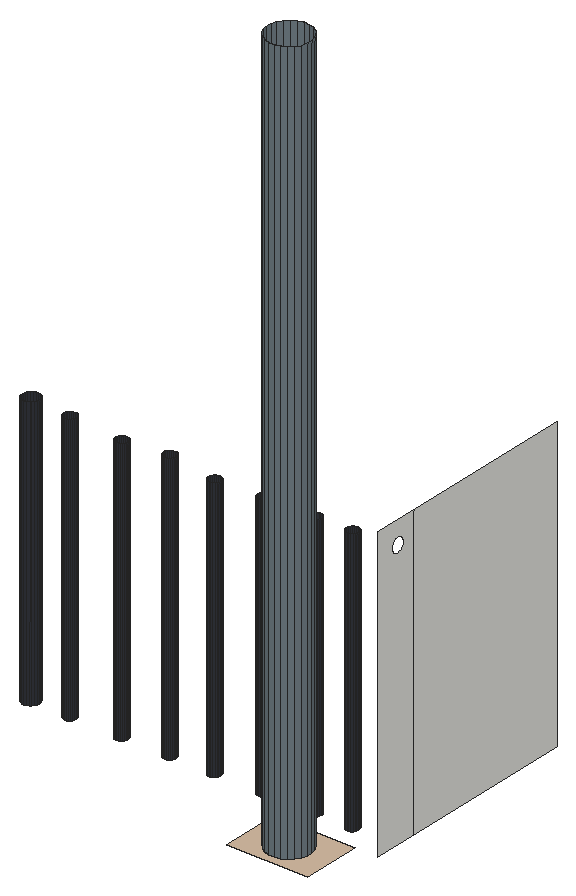
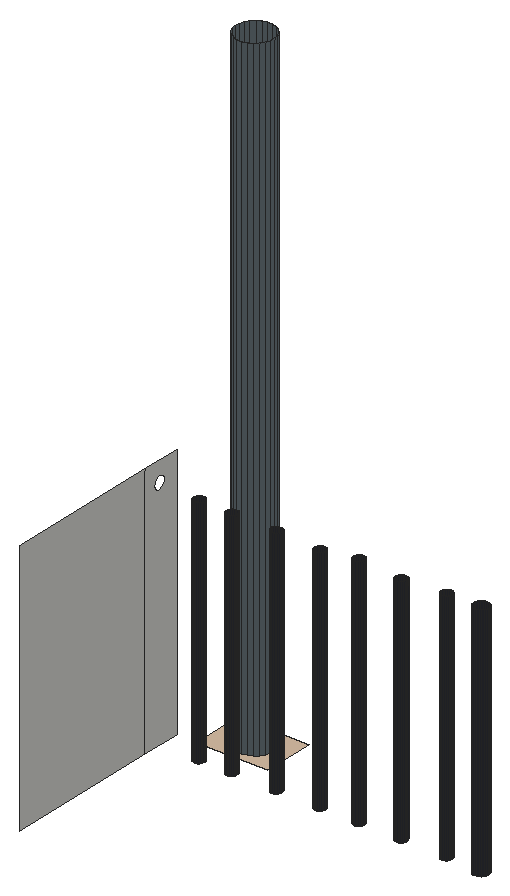
# SketchUp Ruby script. Lengths in inches.
U = 1.inch
M = Sketchup.active_model
def pt(a) = Geom::Point3d.new(a.map { |v| v * U })
def face(e, loops, mat)
  f = e.add_face(loops[0].map { |a| pt(a) })
  loops[1..].each { |l| e.add_face(l.map { |a| pt(a) }).erase! }
  f.material = f.back_material = mat if mat
  f
end
# faces: each face lists its corners as indices into pts; further lists are holes
def faces(e, pts, list, mat = nil) = list.each { |f| face(e, (f[0].is_a?(Array) ? f : [f]).map { |l| l.map { |i| pts[i] } }, mat) }
# xy, xz, yz: faces in a plane at the given z, y or x. An outline is a flat list of corners, or four numbers for a rectangle; further outlines are holes
def ring(l) = l.size == 4 ? [[l[0], l[1]], [l[2], l[1]], [l[2], l[3]], [l[0], l[3]]] : l.each_slice(2).to_a
def flat(e, list, mat, &to3) = list.each { |f| face(e, (f[0].is_a?(Array) ? f : [f]).map { |l| ring(l).map { |u, v| to3.(u, v) } }, mat) }
def xy(e, z, list, mat = nil) = flat(e, list, mat) { |x, y| [x, y, z] }
def xz(e, y, list, mat = nil) = flat(e, list, mat) { |x, z| [x, y, z] }
def yz(e, x, list, mat = nil) = flat(e, list, mat) { |y, z| [x, y, z] }
def lines(e, pts, list) = list.each { |a, b| e.add_line(pt(pts[a]), pt(pts[b])) }
# prism: a flat outline (further loops are holes) pulled along v
def prism(e, loops, v, mat = nil)
  f = face(e, loops, mat); d = Geom::Vector3d.new(v.map { |x| x * U })
  f.pushpull(f.normal.samedirection?(d) ? d.length : -d.length)
end
def box(e, o, s, mat = nil) = prism(e, [[o, [o[0] + s[0], o[1], o[2]], [o[0] + s[0], o[1] + s[1], o[2]], [o[0], o[1] + s[1], o[2]]]], [0, 0, s[2]], mat)
def at(x, y, z, deg = 0) = Geom::Transformation.translation(pt([x, y, z])) * Geom::Transformation.rotation(ORIGIN, Z_AXIS, deg.degrees)
def axes(o, x, y, z) = Geom::Transformation.new([*x, 0, *y, 0, *z, 0, *pt(o).to_a, 1])
def part(name) = M.definitions.add(name)
# library, detail: a bought-in or finely detailed component or shape, given as its bounding box
def library(name, o, s) = part(name).tap { |d| box(d.entities, o, s) }
def detail(e, o, s) = box(e.add_group.entities, o, s)
def put(e, d, t, mat = nil) = e.add_instance(d, t).tap { |i| i.material = mat if mat }
def group(e, t, mat = nil) = e.add_group.tap { |g| g.transformation = t; g.material = mat if mat }.entities
root = M.entities
M.materials.add("[Formica Laminate Dark]").color = [50, 53, 60]
M.materials.add("[Formica Laminate Light]").color = [213, 189, 164]
M.materials.add("[Formica Speckled Grey]").color = [112, 125, 132]
xy(root,160.3,[[376.35,84.16,375.77,84.33,375.25,84.63,374.83,85.07,374.53,85.59,374.38,86.18,374.39,86.78,374.55,87.36,374.86,87.88,375.29,88.3,375.82,88.6,376.4,88.75,377.01,88.74,377.59,88.58,378.11,88.27,378.53,87.84,378.83,87.3125,378.98,86.73,378.97,86.125,378.81,85.54,378.5,85.02,378.07,84.6,377.54,84.31,376.95,84.16],[343.65,91.54,343.41,91.57,343.18,91.66,342.99,91.8125,342.84,92.01,342.75,92.23,342.71,92.47,342.75,92.72,342.84,92.94,342.99,93.14,343.18,93.29,343.41,93.38,343.65,93.41,343.89,93.38,344.12,93.29,344.31,93.14,344.46,92.94,344.56,92.72,344.59,92.47,344.56,92.23,344.46,92.01,344.31,91.8125,344.12,91.66,343.89,91.57],[348.06,91.61,347.88,91.64,347.72,91.7,347.57,91.8125,347.46,91.96,347.4,92.12,347.37,92.3,347.4,92.48,347.46,92.64,347.57,92.79,347.72,92.89,347.88,92.96,348.06,92.99,348.24,92.96,348.4,92.89,348.55,92.79,348.65,92.64,348.72,92.48,348.75,92.3,348.72,92.12,348.65,91.96,348.55,91.8125,348.4,91.7,348.24,91.64],[353.72,91.61,353.54,91.64,353.375,91.7,353.23,91.8125,353.125,91.96,353.06,92.12,353.03,92.3,353.06,92.48,353.125,92.64,353.23,92.79,353.375,92.89,353.54,92.96,353.72,92.99,353.9,92.96,354.0625,92.89,354.21,92.79,354.32,92.64,354.38,92.48,354.41,92.3,354.38,92.12,354.32,91.96,354.21,91.8125,354.0625,91.7,353.9,91.64],[358.97,91.61,358.79,91.64,358.625,91.7,358.48,91.8125,358.375,91.96,358.31,92.12,358.28,92.3,358.31,92.48,358.375,92.64,358.48,92.79,358.625,92.89,358.79,92.96,358.97,92.99,359.15,92.96,359.3125,92.89,359.46,92.79,359.57,92.64,359.63,92.48,359.66,92.3,359.63,92.12,359.57,91.96,359.46,91.8125,359.3125,91.7,359.15,91.64],
  [363.84,91.61,363.67,91.64,363.5,91.7,363.36,91.8125,363.25,91.96,363.18,92.12,363.16,92.3,363.18,92.48,363.25,92.64,363.36,92.79,363.5,92.89,363.67,92.96,363.84,92.99,364.02,92.96,364.1875,92.89,364.33,92.79,364.44,92.64,364.51,92.48,364.53,92.3,364.51,92.12,364.44,91.96,364.33,91.8125,364.1875,91.7,364.02,91.64],[369.28,91.61,369.1,91.64,368.9375,91.7,368.8,91.8125,368.6875,91.96,368.62,92.12,368.59,92.3,368.62,92.48,368.6875,92.64,368.8,92.79,368.9375,92.89,369.1,92.96,369.28,92.99,369.46,92.96,369.625,92.89,369.77,92.79,369.88,92.64,369.95,92.48,369.97,92.3,369.95,92.12,369.88,91.96,369.77,91.8125,369.625,91.7,369.46,91.64],[374.84,91.61,374.67,91.64,374.5,91.7,374.36,91.8125,374.25,91.96,374.18,92.12,374.16,92.3,374.18,92.48,374.25,92.64,374.36,92.79,374.5,92.89,374.67,92.96,374.84,92.99,375.02,92.96,375.1875,92.89,375.33,92.79,375.44,92.64,375.51,92.48,375.53,92.3,375.51,92.12,375.44,91.96,375.33,91.8125,375.1875,91.7,375.02,91.64],[378.93,91.61,378.76,91.64,378.59,91.7,378.45,91.8125,378.34,91.96,378.27,92.12,378.25,92.3,378.27,92.48,378.34,92.64,378.45,92.79,378.59,92.89,378.76,92.96,378.93,92.99,379.11,92.96,379.28,92.89,379.42,92.79,379.53,92.64,379.6,92.48,379.62,92.3,379.6,92.12,379.53,91.96,379.42,91.8125,379.28,91.7,379.11,91.64]])
xy(root,160.3,[[[372.44,83.29,381.28,89.73],[376.35,84.16,375.77,84.33,375.25,84.63,374.83,85.07,374.53,85.59,374.38,86.18,374.39,86.78,374.55,87.36,374.86,87.88,375.29,88.3,375.82,88.6,376.4,88.75,377.01,88.74,377.59,88.58,378.11,88.27,378.53,87.84,378.83,87.3125,378.98,86.73,378.97,86.125,378.81,85.54,378.5,85.02,378.07,84.6,377.54,84.31,376.95,84.16]]],"[Formica Laminate Light]")
xz(root,84.16,[[376.35,160.3,376.95,239.81]],"[Formica Speckled Grey]")
yz(root,383.79,[[[89.73,160.3,94.63,192.125],[92.39,188.79,92.6,188.82,92.8,188.9,92.96,189.03,93.09,189.2,93.18,189.39,93.2,189.6,93.18,189.8125,93.09,190.01,92.96,190.18,92.8,190.31,92.6,190.39,92.39,190.42,92.18,190.39,91.98,190.31,91.82,190.18,91.6875,190.01,91.61,189.8125,91.58,189.6,91.61,189.39,91.6875,189.2,91.82,189.03,91.98,188.9,92.18,188.82]],[94.63,160.3,114.1,192.125]])
p = [[375.77,84.33,160.3],[376.35,84.16,160.3],[376.35,84.16,239.81],[375.77,84.33,239.81],[376.95,84.16,160.3],[377.54,84.31,160.3],
  [377.54,84.31,239.81],[376.95,84.16,239.81],[375.25,84.63,160.3],[375.25,84.63,239.81],[378.07,84.6,160.3],[378.07,84.6,239.81],
  [374.83,85.07,160.3],[374.83,85.07,239.81],[378.5,85.02,160.3],[378.5,85.02,239.81],[378.81,85.54,160.3],[378.81,85.54,239.81],
  [374.53,85.59,160.3],[374.53,85.59,239.81],[378.97,86.125,160.3],[378.97,86.125,239.81],[374.38,86.18,160.3],[374.38,86.18,239.81],
  [378.98,86.73,160.3],[378.98,86.73,239.81],[374.39,86.78,160.3],[374.39,86.78,239.81],[378.83,87.3125,160.3],[378.83,87.3125,239.81],
  [374.55,87.36,160.3],[374.55,87.36,239.81],[378.53,87.84,160.3],[378.53,87.84,239.81],[374.86,87.88,160.3],[374.86,87.88,239.81],
  [378.11,88.27,160.3],[378.11,88.27,239.81],[375.29,88.3,160.3],[375.29,88.3,239.81],[375.82,88.6,160.3],[375.82,88.6,239.81],
  [377.59,88.58,160.3],[377.59,88.58,239.81],[376.4,88.75,160.3],[376.4,88.75,239.81],[377.01,88.74,160.3],[377.01,88.74,239.81],
  [343.41,91.57,160.3],[343.65,91.54,160.3],[343.65,91.54,190.01],[343.41,91.57,190.01],[343.89,91.57,160.3],[343.89,91.57,190.01],
  [343.18,91.66,160.3],[343.18,91.66,190.01],[344.12,91.66,160.3],[344.12,91.66,190.01],[347.72,91.7,160.3],[347.88,91.64,160.3],
  [347.88,91.64,189.8],[347.72,91.7,189.8],[348.06,91.61,160.3],[348.06,91.61,189.8],[348.24,91.64,160.3],[348.24,91.64,189.8],
  [348.4,91.7,160.3],[348.4,91.7,189.8],[353.375,91.7,160.3],[353.54,91.64,160.3],[353.54,91.64,189.42],[353.375,91.7,189.42],
  [353.72,91.61,160.3],[353.72,91.61,189.42],[353.9,91.64,160.3],[353.9,91.64,189.42],[354.0625,91.7,160.3],[354.0625,91.7,189.42],
  [358.625,91.7,160.3],[358.79,91.64,160.3],[358.79,91.64,189.8125],[358.625,91.7,189.8125],[358.97,91.61,160.3],[358.97,91.61,189.8125],
  [359.15,91.64,160.3],[359.15,91.64,189.8125],[359.3125,91.7,160.3],[359.3125,91.7,189.8125],[363.5,91.7,160.3],[363.67,91.64,160.3],
  [363.67,91.64,189.11],[363.5,91.7,189.11],[363.84,91.61,160.3],[363.84,91.61,189.11],[364.02,91.64,160.3],[364.02,91.64,189.11],
  [364.1875,91.7,160.3],[364.1875,91.7,189.11],[368.9375,91.7,160.3],[369.1,91.64,160.3],[369.1,91.64,189.36],[368.9375,91.7,189.36],
  [369.28,91.61,160.3],[369.28,91.61,189.36],[369.46,91.64,160.3],[369.46,91.64,189.36],[369.625,91.7,160.3],[369.625,91.7,189.36],
  [374.5,91.7,160.3],[374.67,91.64,160.3],[374.67,91.64,189.36],[374.5,91.7,189.36],[374.84,91.61,160.3],[374.84,91.61,189.36],
  [375.02,91.64,160.3],[375.02,91.64,189.36],[375.1875,91.7,160.3],[375.1875,91.7,189.36],[378.59,91.7,160.3],[378.76,91.64,160.3],
  [378.76,91.64,189.42],[378.59,91.7,189.42],[378.93,91.61,160.3],[378.93,91.61,189.42],[379.11,91.64,160.3],[379.11,91.64,189.42],
  [379.28,91.7,160.3],[379.28,91.7,189.42],[342.99,91.8125,160.3],[343.15,91.6875,190.01],[342.99,91.8125,190.01],[344.31,91.8125,160.3],
  [344.31,91.8125,190.01],[344.15,91.6875,190.01],[347.57,91.8125,160.3],[347.57,91.8125,189.8],[348.55,91.8125,160.3],[348.55,91.8125,189.8],
  [353.23,91.8125,160.3],[353.23,91.8125,189.42],[354.21,91.8125,160.3],[354.21,91.8125,189.42],[358.48,91.8125,160.3],[358.48,91.8125,189.8125],
  [359.46,91.8125,160.3],[359.46,91.8125,189.8125],[363.36,91.8125,160.3],[363.36,91.8125,189.11],[364.33,91.8125,160.3],[364.33,91.8125,189.11],
  [368.8,91.8125,160.3],[368.8,91.8125,189.36],[369.77,91.8125,160.3],[369.77,91.8125,189.36],[374.36,91.8125,160.3],[374.36,91.8125,189.36],
  [375.33,91.8125,160.3],[375.33,91.8125,189.36],[378.45,91.8125,160.3],[378.45,91.8125,189.42],[379.42,91.8125,160.3],[379.42,91.8125,189.42],
  [342.84,92.01,160.3],[342.84,92.01,190.01],[344.46,92.01,160.3],[344.46,92.01,190.01],[347.46,91.96,160.3],[347.46,91.96,189.8],
  [348.65,91.96,160.3],[348.65,91.96,189.8],[353.125,91.96,160.3],[353.125,91.96,189.42],[354.32,91.96,160.3],[354.32,91.96,189.42],
  [358.375,91.96,160.3],[358.375,91.96,189.8125],[359.57,91.96,160.3],[359.57,91.96,189.8125],[363.25,91.96,160.3],[363.25,91.96,189.11],
  [364.44,91.96,160.3],[364.44,91.96,189.11],[368.6875,91.96,160.3],[368.6875,91.96,189.36],[369.88,91.96,160.3],[369.88,91.96,189.36],
  [374.25,91.96,160.3],[374.25,91.96,189.36],[375.44,91.96,160.3],[375.44,91.96,189.36],[378.34,91.96,160.3],[378.34,91.96,189.42],
  [379.53,91.96,160.3],[379.53,91.96,189.42],[342.75,92.23,160.3],[342.75,92.23,190.01],[344.56,92.23,160.3],[344.56,92.23,190.01],
  [347.4,92.12,160.3],[347.4,92.12,189.8],[348.72,92.12,160.3],[348.72,92.12,189.8],[353.06,92.12,160.3],[353.06,92.12,189.42],
  [354.38,92.12,160.3],[354.38,92.12,189.42],[358.31,92.12,160.3],[358.31,92.12,189.8125],[359.63,92.12,160.3],[359.63,92.12,189.8125],
  [363.18,92.12,160.3],[363.18,92.12,189.11],[364.51,92.12,160.3],[364.51,92.12,189.11],[368.62,92.12,160.3],[368.62,92.12,189.36],
  [369.95,92.12,160.3],[369.95,92.12,189.36],[374.18,92.12,160.3],[374.18,92.12,189.36],[375.51,92.12,160.3],[375.51,92.12,189.36],
  [378.27,92.12,160.3],[378.27,92.12,189.42],[379.6,92.12,160.3],[379.6,92.12,189.42],[347.37,92.3,160.3],[347.37,92.3,189.8],
  [348.75,92.3,160.3],[348.75,92.3,189.8],[353.03,92.3,160.3],[353.03,92.3,189.42],[354.41,92.3,160.3],[354.41,92.3,189.42],
  [358.28,92.3,160.3],[358.28,92.3,189.8125],[359.66,92.3,160.3],[359.66,92.3,189.8125],[363.16,92.3,160.3],[363.16,92.3,189.11],
  [364.53,92.3,160.3],[364.53,92.3,189.11],[368.59,92.3,160.3],[368.59,92.3,189.36],[369.97,92.3,160.3],[369.97,92.3,189.36],
  [374.16,92.3,160.3],[374.16,92.3,189.36],[375.53,92.3,160.3],[375.53,92.3,189.36],[378.25,92.3,160.3],[378.25,92.3,189.42],
  [379.62,92.3,160.3],[379.62,92.3,189.42],[342.71,92.47,160.3],[342.71,92.47,190.01],[344.59,92.47,160.3],[344.59,92.47,190.01],
  [347.4,92.48,160.3],[347.4,92.48,189.8],[348.72,92.48,160.3],[348.72,92.48,189.8],[353.06,92.48,160.3],[353.06,92.48,189.42],
  [354.38,92.48,160.3],[354.38,92.48,189.42],[358.31,92.48,160.3],[358.31,92.48,189.8125],[359.63,92.48,160.3],[359.63,92.48,189.8125],
  [363.18,92.48,160.3],[363.18,92.48,189.11],[364.51,92.48,160.3],[364.51,92.48,189.11],[368.62,92.48,160.3],[368.62,92.48,189.36],
  [369.95,92.48,160.3],[369.95,92.48,189.36],[374.18,92.48,160.3],[374.18,92.48,189.36],[375.51,92.48,160.3],[375.51,92.48,189.36],
  [378.27,92.48,160.3],[378.27,92.48,189.42],[379.6,92.48,160.3],[379.6,92.48,189.42],[342.75,92.72,160.3],[342.75,92.72,190.01],
  [344.56,92.72,160.3],[344.56,92.72,190.01],[347.46,92.64,160.3],[347.46,92.64,189.8],[348.65,92.64,160.3],[348.65,92.64,189.8],
  [353.125,92.64,160.3],[353.125,92.64,189.42],[354.32,92.64,160.3],[354.32,92.64,189.42],[358.375,92.64,160.3],[358.375,92.64,189.8125],
  [359.57,92.64,160.3],[359.57,92.64,189.8125],[363.25,92.64,160.3],[363.25,92.64,189.11],[364.44,92.64,160.3],[364.44,92.64,189.11],
  [368.6875,92.64,160.3],[368.6875,92.64,189.36],[369.88,92.64,160.3],[369.88,92.64,189.36],[374.25,92.64,160.3],[374.25,92.64,189.36],
  [375.44,92.64,160.3],[375.44,92.64,189.36],[378.34,92.64,160.3],[378.34,92.64,189.42],[379.53,92.64,160.3],[379.53,92.64,189.42],
  [347.57,92.79,160.3],[347.57,92.79,189.8],[348.55,92.79,160.3],[348.55,92.79,189.8],[353.23,92.79,160.3],[353.23,92.79,189.42],
  [354.21,92.79,160.3],[354.21,92.79,189.42],[358.48,92.79,160.3],[358.48,92.79,189.8125],[359.46,92.79,160.3],[359.46,92.79,189.8125],
  [363.36,92.79,160.3],[363.36,92.79,189.11],[364.33,92.79,160.3],[364.33,92.79,189.11],[368.8,92.79,160.3],[368.8,92.79,189.36],
  [369.77,92.79,160.3],[369.77,92.79,189.36],[374.36,92.79,160.3],[374.36,92.79,189.36],[375.33,92.79,160.3],[375.33,92.79,189.36],
  [378.45,92.79,160.3],[378.45,92.79,189.42],[379.42,92.79,160.3],[379.42,92.79,189.42],[342.84,92.94,160.3],[342.84,92.94,190.01],
  [344.46,92.94,160.3],[344.46,92.94,190.01],[347.72,92.89,160.3],[347.72,92.89,189.8],[348.4,92.89,160.3],[348.4,92.89,189.8],
  [353.375,92.89,160.3],[353.375,92.89,189.42],[354.0625,92.89,160.3],[354.0625,92.89,189.42],[358.625,92.89,160.3],[358.625,92.89,189.8125],
  [359.3125,92.89,160.3],[359.3125,92.89,189.8125],[363.5,92.89,160.3],[363.5,92.89,189.11],[364.1875,92.89,160.3],[364.1875,92.89,189.11],
  [368.9375,92.89,160.3],[368.9375,92.89,189.36],[369.625,92.89,160.3],[369.625,92.89,189.36],[374.5,92.89,160.3],[374.5,92.89,189.36],
  [375.1875,92.89,160.3],[375.1875,92.89,189.36],[378.59,92.89,160.3],[378.59,92.89,189.42],[379.28,92.89,160.3],[379.28,92.89,189.42],
  [342.99,93.14,160.3],[342.96,93.09,190.01],[342.99,93.14,190.01],[344.31,93.14,160.3],[344.31,93.14,190.01],[344.35,93.09,190.01],
  [347.88,92.96,160.3],[347.88,92.96,189.8],[348.24,92.96,160.3],[348.24,92.96,189.8],[353.54,92.96,160.3],[353.54,92.96,189.42],
  [353.9,92.96,160.3],[353.9,92.96,189.42],[358.79,92.96,160.3],[358.79,92.96,189.8125],[359.15,92.96,160.3],[359.15,92.96,189.8125],
  [363.67,92.96,160.3],[363.67,92.96,189.11],[364.02,92.96,160.3],[364.02,92.96,189.11],[369.1,92.96,160.3],[369.1,92.96,189.36],
  [369.46,92.96,160.3],[369.46,92.96,189.36],[374.67,92.96,160.3],[374.67,92.96,189.36],[375.02,92.96,160.3],[375.02,92.96,189.36],
  [378.76,92.96,160.3],[378.76,92.96,189.42],[379.11,92.96,160.3],[379.11,92.96,189.42],[348.06,92.99,160.3],[348.06,92.99,189.8],
  [353.72,92.99,160.3],[353.72,92.99,189.42],[358.97,92.99,160.3],[358.97,92.99,189.8125],[363.84,92.99,160.3],[363.84,92.99,189.11],
  [369.28,92.99,160.3],[369.28,92.99,189.36],[374.84,92.99,160.3],[374.84,92.99,189.36],[378.93,92.99,160.3],[378.93,92.99,189.42],
  [343.18,93.29,160.3],[343.18,93.29,190.01],[344.12,93.29,160.3],[344.12,93.29,190.01],[343.41,93.38,160.3],[343.41,93.38,190.01],
  [343.89,93.38,160.3],[343.89,93.38,190.01],[343.65,93.41,160.3],[343.65,93.41,190.01]]
faces(root,p,[[0,1,2,3],[4,5,6,7],[8,0,3,9],[5,10,11,6],[12,8,9,13],[10,14,15,11],[14,16,17,15],[18,12,13,19],
  [16,20,21,17],[22,18,19,23],[20,24,25,21],[26,22,23,27],[24,28,29,25],[30,26,27,31],[28,32,33,29],[34,30,31,35],
  [32,36,37,33],[38,34,35,39],[40,38,39,41],[36,42,43,37],[44,40,41,45],[42,46,47,43],[46,44,45,47]],"[Formica Speckled Grey]")
faces(root,p,[[48,49,50,51],[49,52,53,50],[54,48,51,55],[52,56,57,53],[58,59,60,61],[59,62,63,60],[62,64,65,63],[64,66,67,65],
  [68,69,70,71],[69,72,73,70],[72,74,75,73],[74,76,77,75],[78,79,80,81],[79,82,83,80],[82,84,85,83],[84,86,87,85],
  [88,89,90,91],[89,92,93,90],[92,94,95,93],[94,96,97,95],[98,99,100,101],[99,102,103,100],[102,104,105,103],[104,106,107,105],
  [108,109,110,111],[109,112,113,110],[112,114,115,113],[114,116,117,115],[118,119,120,121],[119,122,123,120],[122,124,125,123],[124,126,127,125],
  [128,54,55,129,130],[56,131,132,133,57],[134,58,61,135],[66,136,137,67],[138,68,71,139],[76,140,141,77],[142,78,81,143],[86,144,145,87],
  [146,88,91,147],[96,148,149,97],[150,98,101,151],[106,152,153,107],[154,108,111,155],[116,156,157,117],[158,118,121,159],[126,160,161,127],
  [162,128,130,163],[131,164,165,132],[166,134,135,167],[136,168,169,137],[170,138,139,171],[140,172,173,141],[174,142,143,175],[144,176,177,145],
  [178,146,147,179],[148,180,181,149],[182,150,151,183],[152,184,185,153],[186,154,155,187],[156,188,189,157],[190,158,159,191],[160,192,193,161],
  [194,162,163,195],[164,196,197,165],[198,166,167,199],[168,200,201,169],[202,170,171,203],[172,204,205,173],[206,174,175,207],[176,208,209,177],
  [210,178,179,211],[180,212,213,181],[214,182,183,215],[184,216,217,185],[218,186,187,219],[188,220,221,189],[222,190,191,223],[192,224,225,193],
  [226,198,199,227],[200,228,229,201],[230,202,203,231],[204,232,233,205],[234,206,207,235],[208,236,237,209],[238,210,211,239],[212,240,241,213],
  [242,214,215,243],[216,244,245,217],[246,218,219,247],[220,248,249,221],[250,222,223,251],[224,252,253,225],[254,194,195,255],[196,256,257,197],
  [258,226,227,259],[228,260,261,229],[262,230,231,263],[232,264,265,233],[266,234,235,267],[236,268,269,237],[270,238,239,271],[240,272,273,241],
  [274,242,243,275],[244,276,277,245],[278,246,247,279],[248,280,281,249],[282,250,251,283],[252,284,285,253],[286,254,255,287],[256,288,289,257],
  [290,258,259,291],[260,292,293,261],[294,262,263,295],[264,296,297,265],[298,266,267,299],[268,300,301,269],[302,270,271,303],[272,304,305,273],
  [306,274,275,307],[276,308,309,277],[310,278,279,311],[280,312,313,281],[314,282,283,315],[284,316,317,285],[318,290,291,319],[292,320,321,293],
  [322,294,295,323],[296,324,325,297],[326,298,299,327],[300,328,329,301],[330,302,303,331],[304,332,333,305],[334,306,307,335],[308,336,337,309],
  [338,310,311,339],[312,340,341,313],[342,314,315,343],[316,344,345,317],[346,286,287,347],[288,348,349,289],[350,318,319,351],[320,352,353,321],
  [354,322,323,355],[324,356,357,325],[358,326,327,359],[328,360,361,329],[362,330,331,363],[332,364,365,333],[366,334,335,367],[336,368,369,337],
  [370,338,339,371],[340,372,373,341],[374,342,343,375],[344,376,377,345],[378,346,347,379,380],[348,381,382,383,349],[384,350,351,385],[352,386,387,353],
  [388,354,355,389],[356,390,391,357],[392,358,359,393],[360,394,395,361],[396,362,363,397],[364,398,399,365],[400,366,367,401],[368,402,403,369],
  [404,370,371,405],[372,406,407,373],[408,374,375,409],[376,410,411,377],[412,384,385,413],[386,412,413,387],[414,388,389,415],[390,414,415,391],
  [416,392,393,417],[394,416,417,395],[418,396,397,419],[398,418,419,399],[420,400,401,421],[402,420,421,403],[422,404,405,423],[406,422,423,407],
  [424,408,409,425],[410,424,425,411],[426,378,380,427],[381,428,429,382],[430,426,427,431],[428,432,433,429],[434,430,431,435],[432,434,435,433]],"[Formica Laminate Dark]")
